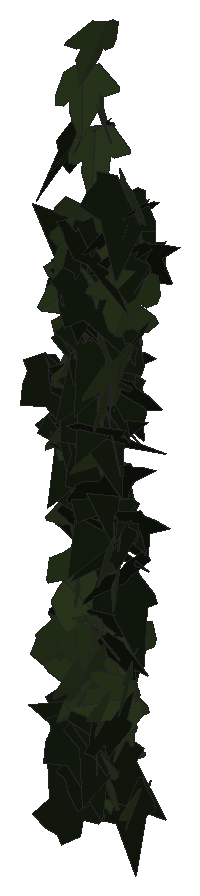
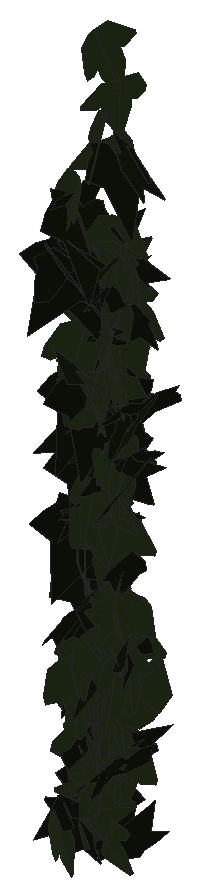
# SketchUp Ruby script. Lengths in inches.
U = 1.inch
M = Sketchup.active_model
def pt(a) = Geom::Point3d.new(a.map { |v| v * U })
def face(e, loops, mat)
  f = e.add_face(loops[0].map { |a| pt(a) })
  loops[1..].each { |l| e.add_face(l.map { |a| pt(a) }).erase! }
  f.material = f.back_material = mat if mat
  f
end
# faces: each face lists its corners as indices into pts; further lists are holes
def faces(e, pts, list, mat = nil) = list.each { |f| face(e, (f[0].is_a?(Array) ? f : [f]).map { |l| l.map { |i| pts[i] } }, mat) }
# xy, xz, yz: faces in a plane at the given z, y or x. An outline is a flat list of corners, or four numbers for a rectangle; further outlines are holes
def ring(l) = l.size == 4 ? [[l[0], l[1]], [l[2], l[1]], [l[2], l[3]], [l[0], l[3]]] : l.each_slice(2).to_a
def flat(e, list, mat, &to3) = list.each { |f| face(e, (f[0].is_a?(Array) ? f : [f]).map { |l| ring(l).map { |u, v| to3.(u, v) } }, mat) }
def xy(e, z, list, mat = nil) = flat(e, list, mat) { |x, y| [x, y, z] }
def xz(e, y, list, mat = nil) = flat(e, list, mat) { |x, z| [x, y, z] }
def yz(e, x, list, mat = nil) = flat(e, list, mat) { |y, z| [x, y, z] }
def lines(e, pts, list) = list.each { |a, b| e.add_line(pt(pts[a]), pt(pts[b])) }
# prism: a flat outline (further loops are holes) pulled along v
def prism(e, loops, v, mat = nil)
  f = face(e, loops, mat); d = Geom::Vector3d.new(v.map { |x| x * U })
  f.pushpull(f.normal.samedirection?(d) ? d.length : -d.length)
end
def box(e, o, s, mat = nil) = prism(e, [[o, [o[0] + s[0], o[1], o[2]], [o[0] + s[0], o[1] + s[1], o[2]], [o[0], o[1] + s[1], o[2]]]], [0, 0, s[2]], mat)
def at(x, y, z, deg = 0) = Geom::Transformation.translation(pt([x, y, z])) * Geom::Transformation.rotation(ORIGIN, Z_AXIS, deg.degrees)
def axes(o, x, y, z) = Geom::Transformation.new([*x, 0, *y, 0, *z, 0, *pt(o).to_a, 1])
def part(name) = M.definitions.add(name)
# library, detail: a bought-in or finely detailed component or shape, given as its bounding box
def library(name, o, s) = part(name).tap { |d| box(d.entities, o, s) }
def detail(e, o, s) = box(e.add_group.entities, o, s)
def put(e, d, t, mat = nil) = e.add_instance(d, t).tap { |i| i.material = mat if mat }
def group(e, t, mat = nil) = e.add_group.tap { |g| g.transformation = t; g.material = mat if mat }.entities
root = M.entities
M.materials.add("efeu1").color = [18, 25, 13]
M.materials.add("efeu2").color = [43, 57, 29]
c1 = part("ivyleaf_10")
p = [[0,0.5,-0.03],[-0.0625,2.02,-0.43],[-0.19,2.01,-0.46],[-0.54,1.05,-0.29],[-0.52,0.625,-0.18],[-0.83,0.76,-0.28],
  [-1.16,0.64,-0.33],[-1.15,0.33,-0.24],[-0.77,-0.39,0.02],[-0.3,-0.51,0.16],[0.04,-0.48,0.23],[-0.02,2.01,-0.4375],
  [-0.06,2.01,-0.43],[0.04,-0.49,0.23],[0.67,-0.49,0.14],[1.38,0.36,-0.2],[1.375,0.51,-0.24],[0.81,0.65,-0.19],
  [0.62,0.59,-0.15],[0.6,1.09,-0.28],[0.5,1.23,-0.31]]
faces(c1.entities,p,[[0,1,2,3,4,5,6,7,8,9,10],[11,12,0,13,14,15,16,17,18,19,20]],"efeu2")
c2 = part("ivyleaf_9")
p = [[1.54,2.16,1.25],[1.36,2.04,1.19],[-0.21,0.99,0.68],[-0.71,1.11,0.82],[-0.85,0.86,0.67],[-0.8,0.17,0.21],
  [-0.9,-0.01,0.1],[-0.67,-0.16,-0.02],[-0.08,-0.08,-0.05],[-0.03,-0.6,-0.4],[0.65,-0.88,-0.66],[0.83,-0.6,-0.49],
  [1.29,-0.42,-0.43],[1.8125,-0.07,-0.26],[1.21,0.44,0.15]]
faces(c2.entities,p,[[0,1,2,3,4,5,6,7,8,9,10,11,12,13,14]],"efeu1")
put(root,c1,axes([510.49,135.18,196.89],[-0.02624,-0.77131,-0.15454],[-0.01385,0.15505,-0.77153],[0.78652,-0.023,-0.01874]))
put(root,c2,axes([509.6875,135.42,195.25],[0.08861,-0.70979,-0.16853],[0.10185,0.17206,-0.73414],[0.77967,0.05819,0.11505]))
put(root,c2,axes([509.25,135.35,200.04],[0.51964,-0.59817,0.07715],[0.10692,-0.00886,-0.78885],[0.59357,0.52526,0.07456]))
put(root,c2,axes([509.69,134.83,194.93],[0.74749,0.12669,0.27796],[0.23284,0.24952,-0.70365],[-0.21869,0.69871,0.20088]))
put(root,c1,axes([509.22,135.23,189.125],[-0.5805,-0.41996,-0.05698],[0.04814,0.03194,-0.70939],[0.45486,-0.53934,0.00236]))
put(root,c2,axes([509.9,135.7,197.01],[-0.60053,-0.50149,0.0585],[-0.05774,-0.02209,-0.78213],[0.50158,-0.60297,-0.02]))
put(root,c2,axes([509.36,135.24,198.93],[0.36749,-0.61019,-0.37263],[-0.09412,0.37404,-0.70532],[0.70876,0.36606,0.09954]))
put(root,c2,axes([509.2,135.1,198.61],[0.5122,-0.34179,-0.49118],[-0.39302,0.3021,-0.60741],[0.49191,0.59726,0.02614]))
put(root,c1,axes([509.23,135.33,198.7],[0.53895,-0.02453,-0.48803],[-0.5019,0.07553,-0.51808],[0.07509,0.68083,0.03989]))
put(root,c1,axes([509.4,135.71,195.56],[-0.05219,0.11112,-0.68139],[0.37843,-0.55391,-0.12458],[-0.60982,-0.35325,-0.01899]))
put(root,c2,axes([509.87,135.86,197.28],[-0.42104,-0.66146,0.09181],[0.02684,-0.12521,-0.779],[0.66727,-0.41234,0.08927]))
put(root,c2,axes([510.01,135.81,196.01],[-0.46198,-0.63034,0.04306],[-0.01429,-0.0429,-0.78138],[0.63165,-0.46199,0.01382]))
put(root,c1,axes([508.76,135.72,199.8125],[0.04362,-0.50816,0.41693],[0.16457,-0.38292,-0.52075],[0.67939,0.12538,0.09937]))
put(root,c2,axes([508.46,135.54,195.93],[0.04888,-0.73348,-0.24714],[0.09454,0.25143,-0.72753],[0.7682,0.01573,0.10526]))
put(root,c2,axes([510.3125,135.05,186.38],[-0.49992,0.5645,0.04604],[0.02098,-0.04131,0.75913],[0.61117,0.46317,0.0116]))
put(root,c1,axes([509.9,135.58,195.79],[-0.41856,-0.6469,0.12752],[0.04523,-0.17886,-0.75888],[0.65779,-0.39933,0.13333]))
put(root,c2,axes([508.87,135.72,202.75],[-0.53852,0.11457,-0.44596],[0.38892,-0.2726,-0.51124],[-0.28023,-0.5985,0.14748]))
put(root,c2,axes([510.26,135.8125,201.29],[-0.08421,-0.71724,0.06179],[-0.01884,-0.05786,-0.75023],[0.77704,-0.07913,-0.01149]))
put(root,c1,axes([510.18,135.28,196.17],[0.27737,-0.64336,-0.34995],[-0.05118,0.35626,-0.69553],[0.73058,0.26922,0.08413]))
put(root,c2,axes([509.09,135.64,186],[0.06061,-0.74439,-0.2178],[0.02192,0.22002,-0.74588],[0.77529,0.05198,0.03811]))
put(root,c2,axes([509.87,135.82,192.5625],[-0.59615,-0.44306,-0.02153],[0.01949,0.0106,-0.73612],[0.47863,-0.55228,0.00315]))
put(root,c1,axes([509.23,135.48,204.37],[0.30027,0.61079,-0.0678],[-0.04229,-0.05379,-0.69779],[-0.66205,0.28046,0.01383]))
put(root,c1,axes([509.1,135.36,197.5625],[-0.54447,-0.08338,-0.49046],[0.50154,0.08222,-0.53141],[0.12639,-0.68542,-0.00408]))
put(root,c1,axes([510.34,135.59,200.49],[0.51106,-0.61334,-0.0575],[-0.03272,0.04758,-0.79834],[0.61516,0.51208,0.0053]))
put(root,c2,axes([510.125,135.09,193.58],[0.33049,0.67449,0.01396],[-0.02542,0.02541,-0.76958],[-0.72815,0.30525,0.0332]))
put(root,c1,axes([510.37,135.63,187.3125],[0.29015,0.00478,-0.68948],[-0.68776,-0.05107,-0.28978],[-0.04892,0.7463,-0.01541]))
put(root,c1,axes([509.99,135.93,191.21],[0.33483,-0.27376,0.646],[0.48879,-0.42248,-0.43239],[0.50333,0.59239,-0.00984]))
put(root,c2,axes([509.14,135.51,194.35],[0.10736,-0.16455,0.68132],[0.70435,-0.14903,-0.14185],[0.18994,0.64564,0.1409]))
put(root,c2,axes([509.26,135.3,199.6],[-0.18658,0.23259,0.63731],[-0.48883,0.41603,-0.29693],[-0.512,-0.48196,0.05124]))
put(root,c1,axes([508.97,135.72,198.66],[-0.45423,0.16734,-0.47349],[0.35541,-0.34426,-0.44776],[-0.38486,-0.51542,0.14534]))
put(root,c1,axes([509.59,135.57,196.53],[-0.42477,-0.67234,-0.00008],[0.0091,-0.00565,-0.7952],[0.67227,-0.42473,0.01071]))
put(root,c2,axes([510.42,135.67,192.1],[-0.69893,0.25948,-0.10469],[0.08368,-0.07675,-0.72382],[-0.2887,-0.65043,0.04365]))
put(root,c1,axes([510.24,135.34,191.79],[0.22862,-0.59011,-0.41865],[-0.07783,0.41645,-0.62951],[0.71933,0.23261,0.06495]))
put(root,c1,axes([509.1875,135.24,190.06],[0.25204,0.48806,0.47827],[0.22459,0.41025,-0.56257],[-0.68854,0.31247,-0.00842]))
put(root,c1,axes([510.52,135.81,198.94],[-0.38394,-0.64843,0.24389],[-0.02431,-0.26606,-0.74563],[0.69235,-0.36892,0.10907]))
put(root,c2,axes([508.79,135.73,198.62],[-0.4359,-0.13605,-0.52571],[0.52154,0.1496,-0.44289],[0.21821,-0.62932,0.00837]))
put(root,c1,axes([509.52,135.81,205.66],[-0.10776,-0.63714,0.22696],[-0.00952,-0.21936,-0.67024],[0.72729,-0.09727,0.02485]))
put(root,c1,axes([509.51,135.62,202.71],[0.28675,0.5976,-0.1081],[-0.04998,-0.09318,-0.68007],[-0.65319,0.26948,0.00458]))
put(root,c1,axes([509.39,135.97,196.1],[0.29711,-0.59237,0.41737],[0.18522,-0.37403,-0.6627],[0.70057,0.35011,-0.0018]))
put(root,c1,axes([509.04,135.93,188.93],[0.02272,-0.20576,-0.61517],[0.41484,-0.46322,0.18179],[-0.53423,-0.36845,0.115]))
put(root,c2,axes([509.4,135.83,193.59],[0.15932,-0.70306,-0.08362],[-0.02514,0.07726,-0.74707],[0.76384,0.14918,-0.00714]))
put(root,c2,axes([509.33,135.77,196.5],[0.36278,-0.69622,-0.03167],[0.05198,0.06264,-0.78148],[0.695,0.35873,0.07498]))
put(root,c1,axes([508.77,136.06,190.36],[0.10394,-0.15547,0.68434],[0.47442,-0.4909,-0.18744],[0.55513,0.44864,0.03205]))
put(root,c1,axes([509.61,135.61,196.67],[0.58371,-0.47287,-0.23227],[-0.14552,0.18846,-0.74938],[0.50634,0.59929,0.05239]))
put(root,c2,axes([510.05,135.4,188.98],[0.69803,0.08845,-0.32089],[-0.33128,-0.03403,-0.67841],[-0.10206,0.71539,0.00741]))
put(root,c2,axes([509.33,135.44,189.44],[0.45524,0.39864,-0.36394],[-0.3328,-0.1798,-0.59903],[-0.4663,0.5175,0.07222]))
put(root,c2,axes([508.86,135.52,191.76],[0.69464,-0.08628,0.30951],[0.31866,-0.03885,-0.6749],[0.10219,0.70763,0.00069]))
put(root,c2,axes([509.02,135.69,183.52],[-0.4542,-0.5059,0.18017],[0.12992,0.12524,0.68408],[-0.56271,0.43726,0.01251]))
put(root,c1,axes([509.02,135.78,196.85],[0.25545,-0.75301,-0.0026],[0.01551,0.00801,-0.79497],[0.75286,0.25534,0.01726]))
put(root,c1,axes([508.92,136.11,186.79],[-0.02735,-0.25974,0.55687],[0.04242,-0.5355,-0.26822],[0.64133,0.02435,0.04149]))
put(root,c1,axes([509.01,135.6875,187.74],[0.06841,-0.73655,-0.10429],[0.00981,0.10561,-0.73947],[0.74383,0.06635,0.01934]))
put(root,c1,axes([509.3,135.53,197.97],[-0.22443,0.62656,0.09239],[-0.02881,0.08474,-0.68652],[-0.68284,-0.2095,-0.00139]))
put(root,c1,axes([509.49,135.72,199.77],[0.59307,-0.02025,-0.39612],[-0.40882,0.05309,-0.57052],[0.05061,0.66619,0.03343]))
put(root,c1,axes([509.22,135.61,192.25],[-0.66352,-0.36756,-0.08633],[0.07033,0.05119,-0.75845],[0.37095,-0.66715,-0.01063]))
put(root,c1,axes([509.87,135.88,187],[0.10712,-0.65928,0.15889],[0.04726,-0.14784,-0.69304],[0.72937,0.10641,0.02157]))
put(root,c1,axes([509.01,135.66,188.79],[-0.65101,-0.04658,0.25724],[-0.26426,-0.04202,-0.62837],[0.06372,-0.6502,0.02218]))
put(root,c1,axes([509.54,135.59,197.49],[-0.57438,0.53944,-0.02356],[0.01644,-0.0169,-0.78798],[-0.5397,-0.57462,0.00106]))
put(root,c2,axes([509.34,136.21,185.63],[-0.12539,-0.63231,0.26867],[-0.03896,-0.256,-0.66851],[0.73666,-0.12117,0.01037]))
put(root,c2,axes([510.42,135.92,199.58],[-0.74772,0.02362,0.1213],[-0.12621,-0.00492,-0.72039],[-0.02427,-0.70208,0.00913]))
put(root,c1,axes([509.14,135.65,200.51],[-0.7242,-0.02042,0.01317],[-0.01357,-0.00342,-0.69769],[0.02212,-0.67067,0.00316]))
put(root,c2,axes([509.17,135.92,195.85],[0.61445,0.27668,0.39341],[-0.35362,-0.17274,0.67379],[0.326,-0.70886,-0.01063]))
put(root,c1,axes([508.37,135.54,187.75],[-0.28984,-0.40496,0.62058],[0.4626,0.42168,0.49122],[-0.57888,0.53973,0.08184]))
put(root,c2,axes([508.98,136.19,194.1875],[-0.51812,-0.56351,0.03808],[-0.01239,-0.04033,-0.76529],[0.56466,-0.51795,0.01815]))
put(root,c2,axes([510.24,135.58,190.8],[-0.11127,0.69567,-0.1353],[0.02812,-0.12765,-0.73135],[-0.76383,-0.10604,-0.00722]))
put(root,c1,axes([509.51,135.76,194.04],[-0.02215,-0.75954,-0.15927],[0.03995,0.15801,-0.75907],[0.77503,-0.02985,0.03458]))
put(root,c2,axes([509.52,136.21,185.86],[-0.11628,-0.01381,0.75707],[-0.69826,-0.29432,-0.11261],[0.29289,-0.70714,0.03209]))
put(root,c2,axes([508.3125,136.04,195.57],[0.40065,-0.65964,0.09574],[0.05669,-0.07757,-0.77174],[0.66414,0.40456,0.00812]))
put(root,c1,axes([510.4,136.05,188.29],[0.40804,-0.63464,0.15423],[0.0809,-0.13134,-0.75449],[0.64809,0.41597,-0.00293]))
put(root,c1,axes([509.79,135.61,196.36],[-0.4717,0.58066,0.2194],[-0.15847,0.15377,-0.74769],[-0.60016,-0.49698,0.02499]))
put(root,c2,axes([508.73,136.24,194.33],[-0.13228,-0.75721,0.00239],[0.00888,-0.00398,-0.76862],[0.75716,-0.13225,0.00943]))
put(root,c1,axes([509.15,135.92,196.18],[-0.2111,-0.75667,0.00177],[0.00035,-0.00193,-0.78557],[0.75668,-0.2111,0.00085]))
put(root,c1,axes([508.75,135.63,186.1],[-0.15196,-0.60983,-0.38522],[0.14735,0.35913,-0.62665],[0.7061,-0.20619,0.04787]))
put(root,c2,axes([509.13,135.64,202.52],[-0.09653,0.66091,-0.05999],[-0.00725,-0.05911,-0.69344],[-0.71646,-0.08845,0.01511]))
put(root,c1,axes([509.49,135.81,193.26],[-0.23269,0.05946,0.63826],[-0.66585,-0.0119,-0.2239],[-0.00909,-0.65032,0.06245]))
put(root,c2,axes([509.36,136.25,194.88],[0.1608,-0.07307,-0.74769],[0.72715,-0.17697,0.17368],[-0.18875,-0.74403,0.03212]))
put(root,c2,axes([509.47,135.84,193.2],[0.24339,-0.61698,-0.40134],[-0.01271,0.41912,-0.65203],[0.73591,0.21129,0.12147]))
put(root,c2,axes([510.29,135.53,200.62],[-0.04163,0.79987,0.00752],[-0.04221,0.00532,-0.79986],[-0.79879,-0.04197,0.04188]))
put(root,c1,axes([509.67,136.03,188.78],[-0.70354,-0.0436,-0.25005],[0.2584,-0.25287,-0.62648],[-0.0536,-0.6467,0.26183]))
put(root,c2,axes([510.27,135.9,196.98],[-0.51803,0.58635,-0.0881],[-0.05022,-0.15996,-0.76929],[-0.5908,-0.50053,0.14264]))
put(root,c2,axes([509.94,135.64,195.94],[0.67058,0.3296,-0.23157],[-0.20559,-0.10669,-0.74719],[-0.3464,0.70137,-0.00483]))
put(root,c1,axes([508.84,135.9,194.56],[-0.12093,-0.75719,-0.14488],[0.03175,0.14163,-0.76673],[0.77027,-0.12472,0.00886]))
put(root,c1,axes([509.2,135.8,196.26],[0.61421,0.48386,0.06294],[-0.08542,0.20625,-0.752],[-0.4804,0.58196,0.21418]))
put(root,c1,axes([508.875,135.65,189.75],[0.40746,0.33267,0.44245],[0.19711,0.4099,-0.50166],[-0.54895,0.3941,0.14828]))
put(root,c1,axes([509.99,136.13,187.3125],[0.54666,-0.20953,0.4164],[0.4182,-0.1088,-0.56833],[0.25158,0.63614,0.03995]))
put(root,c1,axes([509.25,135.96,184.99],[-0.51012,0.23516,-0.27608],[0.26007,-0.11191,-0.5487],[-0.28118,-0.53014,-0.00664]))
put(root,c2,axes([508.99,135.84,195.67],[0.75317,-0.2063,-0.02432],[-0.02205,0.01157,-0.78089],[0.20655,0.75347,0.00533]))
put(root,c1,axes([508.77,136.05,193.4],[0.41976,-0.00607,0.50313],[0.52241,-0.00831,-0.40426],[0.0111,0.62051,-0.0005]))
put(root,c2,axes([509.22,135.67,189.2],[0.64638,-0.00055,-0.40169],[-0.40318,0.18193,-0.60187],[0.10703,0.68868,0.15868]))
put(root,c1,axes([509.59,135.9,188.31],[0.06039,-0.70294,-0.22829],[-0.00523,0.22864,-0.7054],[0.73907,0.05906,0.01366]))
put(root,c1,axes([508.8,135.91,194.125],[0.28966,0.55553,0.08783],[0.03834,0.07664,-0.64156],[-0.60565,0.27054,0.00139]))
put(root,c2,axes([510.08,135.69,192.19],[0.55497,0.46896,-0.09881],[-0.0882,-0.05142,-0.7233],[-0.50919,0.52003,0.01759]))
put(root,c1,axes([509.46,136.24,192.99],[-0.18607,-0.71305,0.19459],[-0.00311,-0.19991,-0.7355],[0.73912,-0.18035,0.04589]))
put(root,c2,axes([508.38,136.33,193.98],[0.24184,-0.72367,0.05841],[0.00965,-0.05835,-0.76295],[0.72596,0.24185,-0.00931]))
put(root,c1,axes([510.28,135.95,201.41],[-0.57317,0.46347,0.00981],[-0.0114,0.00226,-0.73277],[-0.50053,-0.5308,0.00545]))
put(root,c1,axes([509.21,135.83,196.32],[-0.43994,0.61897,0.18759],[-0.1171,0.14689,-0.75932],[-0.63608,-0.45514,0.01004]))
put(root,c1,axes([508.55,135.9375,190.47],[-0.46712,-0.30364,-0.33894],[0.32276,0.13904,-0.5472],[0.35673,-0.52341,0.05127]))
put(root,c2,axes([509.85,136.29,190.12],[0.19833,-0.72895,-0.0819],[-0.01233,0.08151,-0.75539],[0.73343,0.19849,0.00945]))
put(root,c1,axes([509.23,135.85,185.5],[0.50172,-0.40557,-0.37692],[-0.11808,0.41858,-0.60756],[0.54094,0.46753,0.21697]))
put(root,c1,axes([509.52,136.09,187.4],[-0.04074,-0.69166,-0.08807],[-0.00165,0.08489,-0.72037],[0.75257,-0.03726,-0.00635]))
put(root,c2,axes([509.4,135.78,185.19],[-0.05014,-0.18056,-0.77806],[0.27048,0.72969,-0.18677],[0.75155,-0.27466,0.0153]))
put(root,c2,axes([510.04,136.28,184.29],[-0.40295,-0.14715,-0.56913],[0.58414,0.10301,-0.41232],[0.1826,-0.65427,0.06308]))
put(root,c2,axes([510.25,136.1,199.52],[0.002,0.57384,-0.43428],[0.00415,-0.41758,-0.59678],[-0.76646,-0.00076,-0.00436]))
put(root,c2,axes([510.6,136.12,199.51],[-0.62155,0.38213,0.04295],[-0.04221,0.0158,-0.7184],[-0.41295,-0.57677,0.00878]))
put(root,c1,axes([509.43,135.92,203.44],[-0.46348,0.47926,0.20119],[-0.13929,0.14419,-0.66905],[-0.54052,-0.44811,-0.0001]))
put(root,c1,axes([509.64,136.19,186.64],[0.71161,-0.17393,0.10697],[0.13001,0.05612,-0.70332],[0.17527,0.66452,0.08739]))
put(root,c1,axes([509.12,136.47,189.43],[-0.26539,-0.58044,0.37251],[-0.03768,-0.38634,-0.62883],[0.68866,-0.24483,0.10915]))
put(root,c1,axes([509.89,136.08,197.53],[-0.49305,-0.57297,-0.1927],[0.16317,0.1133,-0.75436],[0.58207,-0.5171,0.04824]))
put(root,c2,axes([508.45,136.19,186.39],[0.19595,-0.57614,-0.32871],[-0.00461,0.32686,-0.62218],[0.7097,0.16119,0.08671]))
put(root,c1,axes([509.67,136.29,196.47],[0.63825,-0.26008,-0.03706],[-0.03382,0.01731,-0.67149],[0.28149,0.5918,0.00335]))
put(root,c1,axes([508.73,136.59,185.21],[-0.04492,0.23848,-0.55594],[-0.13588,-0.52702,-0.23435],[-0.61739,0.09864,0.09202]))
put(root,c1,axes([508.99,135.99,185.41],[-0.10265,-0.08244,-0.66456],[0.64931,0.22089,-0.12264],[0.25018,-0.60709,0.04563]))
put(root,c1,axes([508.92,136.28,188.19],[-0.28568,0.5266,-0.1717],[0.07941,-0.14782,-0.61287],[-0.59071,-0.27455,0.00065]))
put(root,c1,axes([509.15,136.47,189.48],[-0.20985,-0.68234,0.19235],[-0.02653,-0.1929,-0.71324],[0.70844,-0.20935,0.03027]))
put(root,c1,axes([508.76,136.09,188.68],[-0.02369,-0.674,-0.33665],[0.06835,0.3335,-0.67251],[0.75029,-0.05166,0.05063]))
put(root,c1,axes([509.01,136.07,185.57],[0.3296,0.45172,0.34125],[0.19985,0.27097,-0.56696],[-0.5689,0.3569,-0.00146]))
put(root,c1,axes([509.17,136.35,184.3125],[0.53369,-0.04532,-0.38529],[-0.39791,0.03896,-0.51607],[0.06439,0.61638,0.00429]))
put(root,c1,axes([508.59,136.6875,194.38],[0.01318,-0.4293,-0.47682],[0.07823,-0.45454,0.44464],[-0.67381,-0.06117,0.0423]))
put(root,c1,axes([509.33,136.16,193.85],[-0.19211,-0.69056,-0.27825],[0.09251,0.26299,-0.71657],[0.73874,-0.21251,0.01738]))
put(root,c1,axes([509.18,136.25,187.46],[0.25372,-0.6628,-0.221],[0.00464,0.23672,-0.7046],[0.69866,0.23912,0.08494]))
put(root,c1,axes([509.29,136.05,195.77],[-0.0583,0.73394,0.26021],[-0.02765,0.25882,-0.73622],[-0.77821,-0.06418,0.00666]))
put(root,c1,axes([510.26,136.51,184.14],[0.17363,-0.6367,0.11935],[0.03587,-0.10997,-0.68293],[0.6978,0.16408,0.00541]))
put(root,c2,axes([509.4,135.99,196.21],[0.30733,0.71573,-0.08509],[-0.02447,-0.08209,-0.77886],[-0.72035,0.30815,-0.00984]))
put(root,c1,axes([509.42,136.36,186.67],[-0.68951,-0.2333,-0.11919],[0.13525,-0.00975,-0.70489],[0.24599,-0.64857,0.05347]))
put(root,c2,axes([510.17,135.99,199.44],[0.467,0.54581,0.13791],[0.08807,0.10457,-0.72419],[-0.6002,0.44003,0.00103]))
put(root,c1,axes([509.76,136.59,188.57],[-0.40148,-0.60587,0.15225],[-0.02803,-0.16333,-0.72387],[0.62408,-0.3971,0.06543]))
